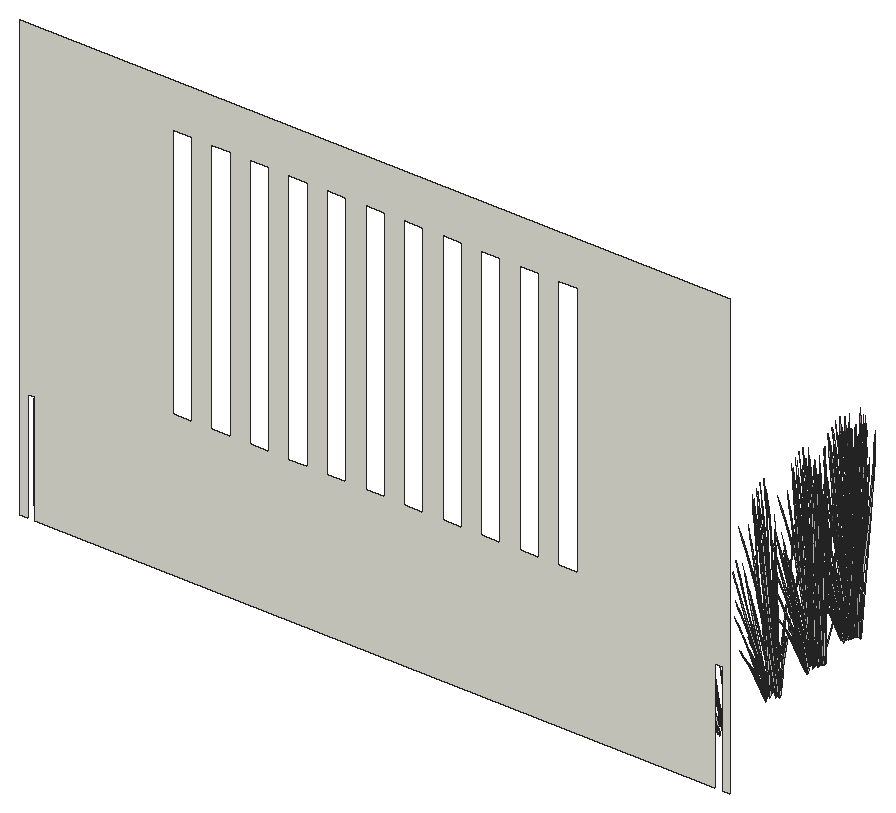
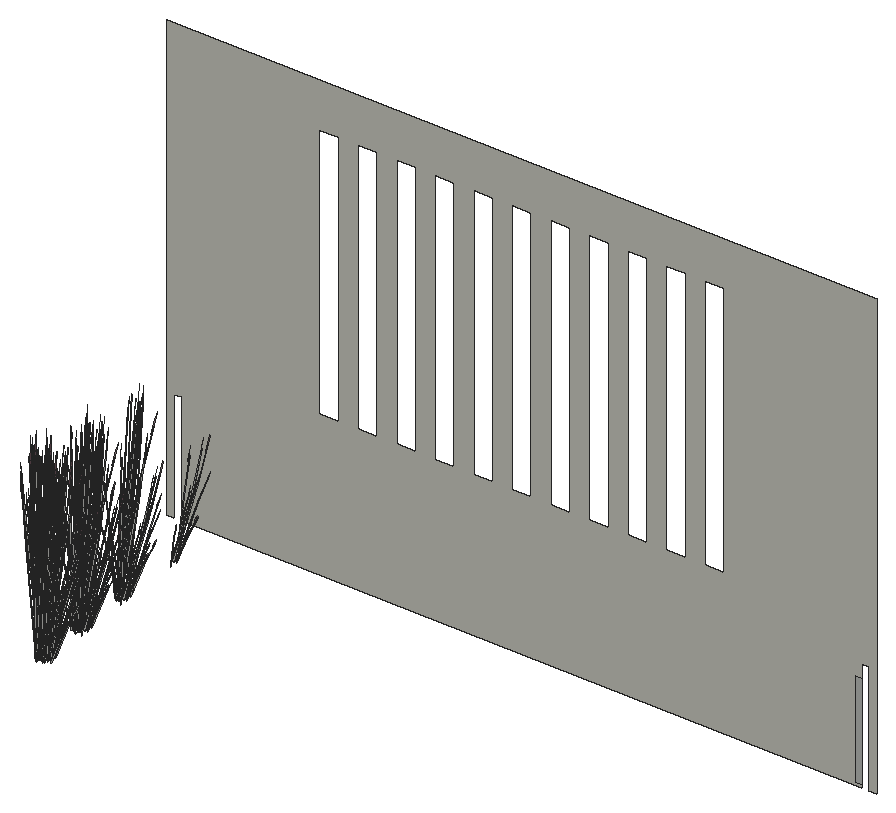
# SketchUp Ruby script. Lengths in inches.
U = 1.inch
M = Sketchup.active_model
def pt(a) = Geom::Point3d.new(a.map { |v| v * U })
def face(e, loops, mat)
  f = e.add_face(loops[0].map { |a| pt(a) })
  loops[1..].each { |l| e.add_face(l.map { |a| pt(a) }).erase! }
  f.material = f.back_material = mat if mat
  f
end
# faces: each face lists its corners as indices into pts; further lists are holes
def faces(e, pts, list, mat = nil) = list.each { |f| face(e, (f[0].is_a?(Array) ? f : [f]).map { |l| l.map { |i| pts[i] } }, mat) }
# xy, xz, yz: faces in a plane at the given z, y or x. An outline is a flat list of corners, or four numbers for a rectangle; further outlines are holes
def ring(l) = l.size == 4 ? [[l[0], l[1]], [l[2], l[1]], [l[2], l[3]], [l[0], l[3]]] : l.each_slice(2).to_a
def flat(e, list, mat, &to3) = list.each { |f| face(e, (f[0].is_a?(Array) ? f : [f]).map { |l| ring(l).map { |u, v| to3.(u, v) } }, mat) }
def xy(e, z, list, mat = nil) = flat(e, list, mat) { |x, y| [x, y, z] }
def xz(e, y, list, mat = nil) = flat(e, list, mat) { |x, z| [x, y, z] }
def yz(e, x, list, mat = nil) = flat(e, list, mat) { |y, z| [x, y, z] }
def lines(e, pts, list) = list.each { |a, b| e.add_line(pt(pts[a]), pt(pts[b])) }
# prism: a flat outline (further loops are holes) pulled along v
def prism(e, loops, v, mat = nil)
  f = face(e, loops, mat); d = Geom::Vector3d.new(v.map { |x| x * U })
  f.pushpull(f.normal.samedirection?(d) ? d.length : -d.length)
end
def box(e, o, s, mat = nil) = prism(e, [[o, [o[0] + s[0], o[1], o[2]], [o[0] + s[0], o[1] + s[1], o[2]], [o[0], o[1] + s[1], o[2]]]], [0, 0, s[2]], mat)
def at(x, y, z, deg = 0) = Geom::Transformation.translation(pt([x, y, z])) * Geom::Transformation.rotation(ORIGIN, Z_AXIS, deg.degrees)
def axes(o, x, y, z) = Geom::Transformation.new([*x, 0, *y, 0, *z, 0, *pt(o).to_a, 1])
def part(name) = M.definitions.add(name)
# library, detail: a bought-in or finely detailed component or shape, given as its bounding box
def library(name, o, s) = part(name).tap { |d| box(d.entities, o, s) }
def detail(e, o, s) = box(e.add_group.entities, o, s)
def put(e, d, t, mat = nil) = e.add_instance(d, t).tap { |i| i.material = mat if mat }
def group(e, t, mat = nil) = e.add_group.tap { |g| g.transformation = t; g.material = mat if mat }.entities
root = M.entities
M.materials.add("D01_Frost_White").color = [238, 238, 227]
M.materials.add("Glass_Basic_01").color = [161, 173, 186]
M.materials["Glass_Basic_01"].alpha = 0.25
M.materials.add("LightPink_Translucent").color = [144, 107, 117]
M.materials["LightPink_Translucent"].alpha = 0.75
c1 = part("blade")
p = [[2.15,0.21,22],[0,0.17,0],[0.09,0.45,0],[2.18,0.31,22],[2.29,0.31,22],[0.38,0.45,0],
  [2.48,0.24,33],[2.49,0.24,33],[2.48,0.22,33]]
faces(c1.entities,p,[[0,1,2,3],[4,5,2,3],[6,3,4,7],[8,0,3,6]])
c2 = part("seeds")
p = [[0.3,-0.1,1.38],[-0.01,-0.03,1.59],[-0.01,-0.03,0.03],[0.14,-0.07,-0.07],[0.29,-0.03,3],[0.15,0.01,3.11]]
faces(c2.entities,p,[[0,1,2,3],[1,0,4,5]],"LightPink_Translucent")
c3 = part("blade with seeds")
put(c3.entities,c1,at(0,0,0))
put(c3.entities,c2,axes([2.4,0.25,30.99],[1.5799,-0.05474,1.17369],[-0.12525,1.92788,0.29478],[-0.07173,-0.02425,1.56792]))
xz(root,178,[[[124,147,124,267,316,267,316,147,314,147,314,177,312,177,312,147,128,147,128,177,126,177,126,147],[269.57,186,274.78,255],[165.22,186,170.43,255],[186.09,186,191.3,255],[196.52,186,201.74,255],[206.96,186,212.17,255],[238.26,186,243.48,255],[248.7,186,253.91,255],[175.65,186,180.87,255],[217.39,186,222.61,255],[227.83,186,233.04,255],[259.13,186,264.35,255]]],"D01_Frost_White")
xz(root,180,[[126,149,128,175]],"Glass_Basic_01")
put(root,c3,axes([300.43,193.49,149.1875],[0.08001,0.13132,1.20808],[-0.18437,0.35694,-0.25981],[-0.18931,-0.08532,0.51652]))
put(root,c3,axes([300.76,193.37,151.21],[-0.40965,-0.01136,-0.60019],[0.02751,-0.47821,0.07243],[-0.17355,-0.05047,0.84903]))
put(root,c3,axes([300.625,193.47,150.95],[-0.29757,0.31243,-0.43168],[-0.2606,-0.33005,-0.33437],[-0.15119,-0.04754,0.82598]))
put(root,c3,axes([299.95,193.88,149.34],[0.26163,-0.03375,0.97034],[-0.16596,0.29737,0.71294],[-0.12929,-0.04461,0.21373]))
put(root,c3,axes([300.14,194.37,148.26],[0.01039,0.07433,1.48974],[-0.20952,0.38819,-0.22758],[-0.14882,-0.01957,0.25375]))
put(root,c3,axes([301.14,194.14,149.82],[0.11649,-0.06823,1.49584],[0.04017,0.47639,0.11706],[-0.25231,0.06321,0.53462]))
put(root,c3,axes([300.34,194.4,150.95],[-0.11102,0.42903,-0.43168],[-0.38064,-0.14706,-0.33437],[-0.15325,0.03934,0.82598]))
put(root,c3,axes([299.88,195.4,149.1875],[0.14242,0.03872,1.20808],[0.09179,0.39548,-0.25981],[-0.19345,0.07403,0.51652]))
put(root,c3,axes([299.58,196.23,149.34],[0.17079,-0.21377,0.97034],[0.06739,0.33841,0.71294],[-0.12342,0.0606,0.21373]))
put(root,c3,axes([300.03,196.45,148.26],[0.05497,0.04712,1.48974],[0.09321,0.43661,-0.22758],[-0.12183,0.0931,0.25375]))
put(root,c3,axes([299.08,211.59,149.1875],[-0.02482,0.15429,1.20808],[-0.36278,0.12916,-0.25981],[-0.0848,-0.19943,0.51652]))
put(root,c3,axes([298.96,211.35,149.34],[0.21377,0.16416,0.97034],[-0.31132,0.09868,0.71294],[-0.06661,-0.12616,0.21373]))
put(root,c3,axes([299.47,212.22,151.21],[-0.34944,-0.22798,-0.60019],[0.24834,-0.39949,0.07243],[-0.1266,-0.13612,0.84903]))
put(root,c3,axes([298.79,211.84,148.26],[-0.0397,0.06213,1.48974],[-0.40116,0.13396,-0.22758],[-0.09691,-0.12186,0.25375]))
put(root,c3,axes([299.31,212.23,150.95],[-0.40438,0.11212,-0.43168],[-0.07074,-0.4246,-0.33437],[-0.10862,-0.12168,0.82598]))
put(root,c3,axes([300.31,214.8,149.81],[0.35414,0.19019,1.27785],[-0.34693,0.40974,0.50532],[-0.1554,-0.24285,1.07126]))
put(root,c3,axes([298.54,212.08,148.8],[-0.11822,0.38513,-0.03288],[-0.36385,-0.11847,-0.1491],[-0.05524,-0.06299,0.4918]))
put(root,c3,axes([298.34,213.84,149],[-0.51243,0,0],[0,-0.52715,-0.43598],[0,-0.12006,1.38303]))
put(root,c3,axes([298.43,212.9,149.1875],[0.08001,0.13132,1.20808],[-0.18437,0.35694,-0.25981],[-0.18931,-0.08532,0.51652]))
put(root,c3,axes([298.76,212.78,151.21],[-0.40965,-0.01136,-0.60019],[0.02751,-0.47821,0.07243],[-0.17355,-0.05047,0.84903]))
put(root,c3,axes([298.74,213.7,148.97],[-0.38118,0.39654,0.25983],[-0.38142,-0.39237,-0.30828],[-0.01331,-0.11261,1.39295]))
put(root,c3,axes([299.77,214.53,149.06],[0.10862,-0.55889,-0.19793],[0.515,0.09742,0.43313],[-0.08999,-0.07718,1.32161]))
put(root,c3,axes([298.625,212.875,150.95],[-0.29757,0.31243,-0.43168],[-0.2606,-0.33005,-0.33437],[-0.15119,-0.04754,0.82598]))
put(root,c3,axes([297.95,213.29,149.34],[0.26163,-0.03375,0.97034],[-0.16596,0.29737,0.71294],[-0.12929,-0.04461,0.21373]))
put(root,c3,axes([299.74,214.3,148.87],[-0.24618,-0.39589,-0.37796],[0.37289,-0.27878,0.1819],[-0.07967,-0.04899,1.2135]))
put(root,c3,axes([299.51,214.45,148.74],[-0.42629,-0.07733,-0.52676],[0.08996,-0.47699,-0.13825],[-0.12722,-0.0578,1.16273]))
put(root,c3,axes([298.14,213.78,148.26],[0.01039,0.07433,1.48974],[-0.20952,0.38819,-0.22758],[-0.14882,-0.01957,0.25375]))
put(root,c3,axes([299.0625,215.18,148.71],[-0.09626,-0.41098,-0.2617],[0.38233,-0.1167,0.2617],[-0.07708,-0.04739,1.17405]))
put(root,c3,axes([298.96,215.35,148.7],[-0.38354,-0.23583,-0.41945],[0.22925,-0.42288,0],[-0.08735,-0.05371,1.33059]))
put(root,c3,axes([300,214.52,149.25],[-0.41376,0.31314,-0.2458],[-0.27514,-0.44246,-0.42242],[-0.10209,-0.04493,1.34921]))
put(root,c3,axes([299.14,213.54,149.82],[0.11649,-0.06823,1.49584],[0.04017,0.47639,0.11706],[-0.25231,0.06321,0.53462]))
put(root,c3,axes([300.46,214.66,149.08],[-0.40016,-0.37963,-0.21282],[0.33672,-0.42629,0.46574],[-0.10776,0.04441,1.42109]))
put(root,c3,axes([299.41,215.39,149.09],[0.38354,0.23583,0.41945],[-0.22925,0.42288,0],[-0.08735,-0.05371,1.33059]))
put(root,c3,axes([298.34,213.8,150.95],[-0.11102,0.42903,-0.43168],[-0.38064,-0.14706,-0.33437],[-0.15325,0.03934,0.82598]))
put(root,c3,axes([299.1875,215.64,149],[-0.25622,0.47263,0],[-0.42866,-0.26357,-0.43598],[-0.09763,-0.06003,1.38303]))
put(root,c3,axes([300.26,214.58,148.87],[-0.44501,0.02912,-0.37796],[-0.04024,-0.48332,0.1819],[-0.07967,0.04899,1.2135]))
put(root,c3,axes([297.88,214.8125,149.1875],[0.14242,0.03872,1.20808],[0.09179,0.39548,-0.25981],[-0.19345,0.07403,0.51652]))
put(root,c3,axes([297.58,215.64,149.34],[0.17079,-0.21377,0.97034],[0.06739,0.33841,0.71294],[-0.12342,0.0606,0.21373]))
put(root,c3,axes([300.27,214.86,148.74],[-0.27603,0.35451,-0.52676],[-0.34289,-0.32147,-0.13825],[-0.11061,0.08844,1.16273]))
put(root,c3,axes([298.52,214.76,150.95],[0.10528,0.43067,-0.43168],[-0.39868,0.07534,-0.33437],[-0.11425,0.11568,0.82598]))
put(root,c3,axes([298.03,215.86,148.26],[0.05497,0.04712,1.48974],[0.09321,0.43661,-0.22758],[-0.12183,0.0931,0.25375]))
put(root,c3,axes([299.03,216.57,149.34],[-0.01061,-0.28045,0.97034],[0.26501,0.20003,0.71294],[-0.05212,0.13367,0.21373]))
put(root,c3,axes([299.04,215.34,151.51],[-0.01066,0.43628,-0.66621],[-0.44902,-0.0293,0.0804],[-0.04739,0.18483,0.94242]))
put(root,c3,axes([298.72,216.32,149.1875],[0.12932,-0.07441,1.20808],[0.31929,0.22435,-0.25981],[-0.09503,0.19413,0.51652]))
put(root,c3,axes([298.89,215.96,149.84],[0.009,-0.24349,1.30391],[0.40497,0.12861,0.18019],[-0.03509,0.2595,0.61571]))
put(root,c3,axes([298.45,227.71,151.21],[-0.19559,-0.38351,-0.60019],[0.40262,-0.21373,0.07243],[-0.04574,-0.1853,0.84903]))
put(root,c3,axes([297.18,227.2,149.1875],[-0.02482,0.15429,1.20808],[-0.36278,0.12916,-0.25981],[-0.0848,-0.19943,0.51652]))
put(root,c3,axes([298.11,226.86,148.26],[-0.06874,0.01699,1.48974],[-0.38012,-0.19128,-0.22758],[0.00638,-0.15955,0.25375]))
put(root,c3,axes([298.3,227.63,150.95],[-0.40284,-0.11824,-0.43168],[0.13808,-0.40538,-0.33437],[-0.03694,-0.16321,0.82598]))
put(root,c3,axes([297.05,226.95,149.34],[0.21377,0.16416,0.97034],[-0.31132,0.09868,0.71294],[-0.06661,-0.12616,0.21373]))
put(root,c3,axes([297.57,227.82,151.21],[-0.34944,-0.22798,-0.60019],[0.24834,-0.39949,0.07243],[-0.1266,-0.13612,0.84903]))
put(root,c3,axes([296.88,227.44,148.26],[-0.0397,0.06213,1.48974],[-0.40116,0.13396,-0.22758],[-0.09691,-0.12186,0.25375]))
put(root,c3,axes([297.55,229.15,148.77],[-0.1683,-0.48366,-0.58997],[0.48479,-0.17419,-0.15484],[-0.0186,-0.16378,1.30225]))
put(root,c3,axes([297.41,227.83,150.95],[-0.40438,0.11212,-0.43168],[-0.07074,-0.4246,-0.33437],[-0.10862,-0.12168,0.82598]))
put(root,c3,axes([298.04,227.19,148.8],[-0.28319,0.27058,-0.03288],[-0.25948,-0.29635,-0.1491],[-0.01827,-0.08397,0.4918]))
put(root,c3,axes([298.41,230.4,149.81],[0.35414,0.19019,1.27785],[-0.34693,0.40974,0.50532],[-0.1554,-0.24285,1.07126]))
put(root,c3,axes([296.55,229.08,148.7],[0,-0.47166,-0.41945],[0.45849,0,0],[0,-0.10742,1.33059]))
put(root,c3,axes([297.8,229.28,148.87],[0.19883,-0.425,-0.37796],[0.41314,0.20454,0.1819],[0,-0.09797,1.2135]))
put(root,c3,axes([296.75,229.09,148.71],[0.28606,-0.29428,-0.2617],[0.28606,0.29428,0.2617],[0,-0.09479,1.17405]))
put(root,c3,axes([296.64,227.68,148.8],[-0.11822,0.38513,-0.03288],[-0.36385,-0.11847,-0.1491],[-0.05524,-0.06299,0.4918]))
put(root,c3,axes([297.75,229.63,149.25],[-0.46151,-0.22505,-0.2458],[0.22222,-0.475,-0.42242],[-0.0145,-0.11662,1.34921]))
put(root,c3,axes([296.44,229.44,149],[-0.51243,0,0],[0,-0.52715,-0.43598],[0,-0.12006,1.38303]))
put(root,c3,axes([296.53,228.5,149.1875],[0.08001,0.13132,1.20808],[-0.18437,0.35694,-0.25981],[-0.18931,-0.08532,0.51652]))
put(root,c3,axes([296.86,228.38,151.21],[-0.40965,-0.01136,-0.60019],[0.02751,-0.47821,0.07243],[-0.17355,-0.05047,0.84903]))
put(root,c3,axes([296.84,229.3,148.97],[-0.38118,0.39654,0.25983],[-0.38142,-0.39237,-0.30828],[-0.01331,-0.11261,1.39295]))
put(root,c3,axes([297.87,230.13,149.06],[0.10862,-0.55889,-0.19793],[0.515,0.09742,0.43313],[-0.08999,-0.07718,1.32161]))
put(root,c3,axes([296.72,228.48,150.95],[-0.29757,0.31243,-0.43168],[-0.2606,-0.33005,-0.33437],[-0.15119,-0.04754,0.82598]))
put(root,c3,axes([296.05,228.89,149.34],[0.26163,-0.03375,0.97034],[-0.16596,0.29737,0.71294],[-0.12929,-0.04461,0.21373]))
put(root,c3,axes([296.75,229.52,149.09],[0,0.47166,0.41945],[-0.45849,0,0],[0,-0.10742,1.33059]))
put(root,c3,axes([297.83,229.9,148.87],[-0.24618,-0.39589,-0.37796],[0.37289,-0.27878,0.1819],[-0.07967,-0.04899,1.2135]))
put(root,c3,axes([297.88,229.34,148.99],[0.17817,0.52741,0.38653],[-0.50909,0.1834,0.15168],[0.00622,-0.09691,1.34202]))
put(root,c3,axes([297.8,229.76,149.3],[-0.19883,0.425,0.37796],[-0.41314,-0.20454,-0.1819],[0,-0.09797,1.2135]))
put(root,c3,axes([297.61,230.05,148.74],[-0.42629,-0.07733,-0.52676],[0.08996,-0.47699,-0.13825],[-0.12722,-0.0578,1.16273]))
put(root,c3,axes([298.65,229.81,148.94],[-0.38118,-0.40596,-0.0518],[0.38142,-0.40621,0],[-0.01331,-0.01418,1.48322]))
put(root,c3,axes([297.93,229.86,148.99],[0.51796,0.09937,0.38653],[-0.10541,0.56124,0.15168],[-0.07569,-0.05419,1.34202]))
put(root,c3,axes([296.24,229.38,148.26],[0.01039,0.07433,1.48974],[-0.20952,0.38819,-0.22758],[-0.14882,-0.01957,0.25375]))
put(root,c3,axes([297.16,230.78,148.71],[-0.09626,-0.41098,-0.2617],[0.38233,-0.1167,0.2617],[-0.07708,-0.04739,1.17405]))
put(root,c3,axes([297.65,230.76,149.09],[0.44036,-0.12519,0.14904],[0.10874,0.46588,0.29641],[-0.03927,-0.06788,1.35512]))
put(root,c3,axes([297.05,230.96,148.7],[-0.38354,-0.23583,-0.41945],[0.22925,-0.42288,0],[-0.08735,-0.05371,1.33059]))
put(root,c3,axes([298.1,230.125,149.25],[-0.41376,0.31314,-0.2458],[-0.27514,-0.44246,-0.42242],[-0.10209,-0.04493,1.34921]))
put(root,c3,axes([298.3125,230.65,148.86],[-0.13371,-0.40664,0],[0.38182,-0.1424,0],[0,0,1.30413]))
put(root,c3,axes([298.06,230.26,149.21],[-0.07906,0.42093,0.12232],[-0.38625,-0.07307,-0.3493],[-0.07029,-0.04322,1.07074]))
put(root,c3,axes([298.96,230.78,149.09],[0.11838,-0.46875,0.14904],[0.43321,0.13265,0.29641],[-0.07483,0.00228,1.35512]))
put(root,c3,axes([297.24,229.15,149.82],[0.11649,-0.06823,1.49584],[0.04017,0.47639,0.11706],[-0.25231,0.06321,0.53462]))
put(root,c3,axes([298.22,230.83,148.86],[-0.41314,-0.21175,0],[0.19883,-0.43999,0],[0,0,1.37455]))
put(root,c3,axes([298.5625,230.27,149.08],[-0.40016,-0.37963,-0.21282],[0.33672,-0.42629,0.46574],[-0.10776,0.04441,1.42109]))
put(root,c3,axes([297.51,230.99,149.09],[0.38354,0.23583,0.41945],[-0.22925,0.42288,0],[-0.08735,-0.05371,1.33059]))
put(root,c3,axes([296.43,229.41,150.95],[-0.11102,0.42903,-0.43168],[-0.38064,-0.14706,-0.33437],[-0.15325,0.03934,0.82598]))
put(root,c3,axes([297.29,231.24,149],[-0.25622,0.47263,0],[-0.42866,-0.26357,-0.43598],[-0.09763,-0.06003,1.38303]))
put(root,c3,axes([298.75,229.95,149.3],[0.44501,-0.02912,0.37796],[0.04024,0.48332,-0.1819],[-0.07967,0.04899,1.2135]))
put(root,c3,axes([298.36,230.1875,148.87],[-0.44501,0.02912,-0.37796],[-0.04024,-0.48332,0.1819],[-0.07967,0.04899,1.2135]))
put(root,c3,axes([298.85,231.31,148.85],[-0.25302,-0.47428,-0.04344],[0.42866,-0.26357,0.43598],[-0.10563,0.04516,1.38235]))
put(root,c3,axes([298.76,230.16,149.21],[0.30276,0.28338,0.12232],[-0.25254,0.31972,-0.3493],[-0.07029,0.04322,1.07074]))
put(root,c3,axes([299.08,231.03,149.09],[0.38354,-0.23583,0.41945],[0.22925,0.42288,0],[-0.08735,0.05371,1.33059]))
put(root,c3,axes([298.74,231.25,148.71],[-0.38233,-0.1167,-0.2617],[0.09626,-0.41098,0.2617],[-0.07708,0.04739,1.17405]))
put(root,c3,axes([295.98,230.41,149.1875],[0.14242,0.03872,1.20808],[0.09179,0.39548,-0.25981],[-0.19345,0.07403,0.51652]))
put(root,c3,axes([295.68,231.24,149.34],[0.17079,-0.21377,0.97034],[0.06739,0.33841,0.71294],[-0.12342,0.0606,0.21373]))
put(root,c3,axes([298.67,230.05,149.25],[0.04775,0.53819,-0.2458],[-0.49736,0.03254,-0.42242],[-0.08758,0.07169,1.34921]))
put(root,c3,axes([298.37,230.47,148.74],[-0.27603,0.35451,-0.52676],[-0.34289,-0.32147,-0.13825],[-0.11061,0.08844,1.16273]))
put(root,c3,axes([298.86,231.0625,148.97],[0.51304,0.1533,0.25983],[-0.12835,0.54797,-0.30828],[-0.08491,0.06858,1.39295]))
put(root,c3,axes([298.83,231.43,148.7],[-0.38354,0.23583,-0.41945],[-0.22925,-0.42288,0],[-0.08735,0.05371,1.33059]))
put(root,c3,axes([296.62,230.36,150.95],[0.10528,0.43067,-0.43168],[-0.39868,0.07534,-0.33437],[-0.11425,0.11568,0.82598]))
put(root,c3,axes([299.17,231.36,149],[0.25622,0.47263,0],[-0.42866,0.26357,-0.43598],[-0.09763,0.06003,1.38303]))
put(root,c3,axes([298.96,229.49,149.4],[-0.01119,-0.44408,1.19347],[0.50665,0.11511,0.50532],[-0.11983,0.243,1.12654]))
put(root,c3,axes([296.13,231.46,148.26],[0.05497,0.04712,1.48974],[0.09321,0.43661,-0.22758],[-0.12183,0.0931,0.25375]))
put(root,c3,axes([297.13,232.17,149.34],[-0.01061,-0.28045,0.97034],[0.26501,0.20003,0.71294],[-0.05212,0.13367,0.21373]))
put(root,c3,axes([297.83,231.5,148.26],[0.06632,-0.02567,1.48974],[0.39894,0.14126,-0.22758],[0.01167,0.15921,0.25375]))
put(root,c3,axes([297.23,231.09,151.23],[0.29336,0.31691,-0.47917],[-0.3099,0.27755,-0.37115],[-0.04464,0.16102,0.91684]))
put(root,c3,axes([296.91,231.57,149.38],[0.37228,-0.08352,0.05498],[0.08559,0.3365,-0.7291],[-0.0236,0.17034,0.65354]))
put(root,c3,axes([297.14,230.95,151.51],[-0.01066,0.43628,-0.66621],[-0.44902,-0.0293,0.0804],[-0.04739,0.18483,0.94242]))
put(root,c3,axes([296.82,231.92,149.1875],[0.12932,-0.07441,1.20808],[0.31929,0.22435,-0.25981],[-0.09503,0.19413,0.51652]))
put(root,c3,axes([296.99,231.5625,149.84],[0.009,-0.24349,1.30391],[0.40497,0.12861,0.18019],[-0.03509,0.2595,0.61571]))
put(root,c3,axes([296.75,242.54,149.1875],[-0.11649,0.09547,1.20808],[-0.34886,-0.1671,-0.25981],[0.06467,-0.20781,0.51652]))
put(root,c3,axes([296.22,242.87,151.21],[-0.19559,-0.38351,-0.60019],[0.40262,-0.21373,0.07243],[-0.04574,-0.1853,0.84903]))
put(root,c3,axes([294.95,242.36,149.1875],[-0.02482,0.15429,1.20808],[-0.36278,0.12916,-0.25981],[-0.0848,-0.19943,0.51652]))
put(root,c3,axes([295.88,242.02,148.26],[-0.06874,0.01699,1.48974],[-0.38012,-0.19128,-0.22758],[0.00638,-0.15955,0.25375]))
put(root,c3,axes([297.03,243.25,151.21],[0.01066,-0.43628,-0.60019],[0.44902,0.0293,0.07243],[0.04739,-0.18483,0.84903]))
put(root,c3,axes([296.07,242.79,150.95],[-0.40284,-0.11824,-0.43168],[0.13808,-0.40538,-0.33437],[-0.03694,-0.16321,0.82598]))
put(root,c3,axes([296.32,241.78,149.34],[0.05257,0.27504,0.97034],[-0.29163,-0.15233,0.71294],[0.03138,-0.14083,0.21373]))
put(root,c3,axes([296.94,243.1,150.95],[-0.29336,-0.31691,-0.43168],[0.3099,-0.27755,-0.33437],[0.04464,-0.16102,0.82598]))
put(root,c3,axes([294.82,242.11,149.34],[0.21377,0.16416,0.97034],[-0.31132,0.09868,0.71294],[-0.06661,-0.12616,0.21373]))
put(root,c3,axes([295.34,242.98,151.21],[-0.34944,-0.22798,-0.60019],[0.24834,-0.39949,0.07243],[-0.1266,-0.13612,0.84903]))
put(root,c3,axes([294.65,242.6,148.26],[-0.0397,0.06213,1.48974],[-0.40116,0.13396,-0.22758],[-0.09691,-0.12186,0.25375]))
put(root,c3,axes([295.32,244.3125,148.77],[-0.1683,-0.48366,-0.58997],[0.48479,-0.17419,-0.15484],[-0.0186,-0.16378,1.30225]))
put(root,c3,axes([295.18,242.99,150.95],[-0.40438,0.11212,-0.43168],[-0.07074,-0.4246,-0.33437],[-0.10862,-0.12168,0.82598]))
put(root,c3,axes([295.25,242.92,149],[-0.25622,-0.47263,0],[0.42866,-0.26357,-0.43598],[0.09763,-0.06003,1.38303]))
put(root,c3,axes([295.8125,242.35,148.8],[-0.28319,0.27058,-0.03288],[-0.25948,-0.29635,-0.1491],[-0.01827,-0.08397,0.4918]))
put(root,c3,axes([296.18,245.56,149.81],[0.35414,0.19019,1.27785],[-0.34693,0.40974,0.50532],[-0.1554,-0.24285,1.07126]))
put(root,c3,axes([294.32,244.24,148.7],[0,-0.47166,-0.41945],[0.45849,0,0],[0,-0.10742,1.33059]))
put(root,c3,axes([295.6,242.85,148.7],[0.38354,-0.23583,-0.41945],[0.22925,0.42288,0],[0.08735,-0.05371,1.33059]))
put(root,c3,axes([295.57,244.4375,148.87],[0.19883,-0.425,-0.37796],[0.41314,0.20454,0.1819],[0,-0.09797,1.2135]))
put(root,c3,axes([295.75,244.23,149.25],[-0.04775,-0.53819,-0.2458],[0.49736,-0.03254,-0.42242],[0.08758,-0.07169,1.34921]))
put(root,c3,axes([294.52,244.25,148.71],[0.28606,-0.29428,-0.2617],[0.28606,0.29428,0.2617],[0,-0.09479,1.17405]))
put(root,c3,axes([294.4,242.84,148.8],[-0.11822,0.38513,-0.03288],[-0.36385,-0.11847,-0.1491],[-0.05524,-0.06299,0.4918]))
put(root,c3,axes([295.52,244.79,149.25],[-0.46151,-0.22505,-0.2458],[0.22222,-0.475,-0.42242],[-0.0145,-0.11662,1.34921]))
put(root,c3,axes([294.21,244.6,149],[-0.51243,0,0],[0,-0.52715,-0.43598],[0,-0.12006,1.38303]))
put(root,c3,axes([294.3,243.66,149.1875],[0.08001,0.13132,1.20808],[-0.18437,0.35694,-0.25981],[-0.18931,-0.08532,0.51652]))
put(root,c3,axes([295.6875,243.03,148.71],[0.38233,0.1167,-0.2617],[-0.09626,0.41098,0.2617],[0.07708,-0.04739,1.17405]))
put(root,c3,axes([294.625,243.54,151.21],[-0.40965,-0.01136,-0.60019],[0.02751,-0.47821,0.07243],[-0.17355,-0.05047,0.84903]))
put(root,c3,axes([294.61,244.46,148.97],[-0.38118,0.39654,0.25983],[-0.38142,-0.39237,-0.30828],[-0.01331,-0.11261,1.39295]))
put(root,c3,axes([295.82,244.65,149.06],[0.46174,0.2286,0.2033],[-0.22222,0.475,0.42242],[0,-0.1095,1.35626]))
put(root,c3,axes([295.64,245.29,149.06],[0.10862,-0.55889,-0.19793],[0.515,0.09742,0.43313],[-0.08999,-0.07718,1.32161]))
put(root,c3,axes([294.49,243.64,150.95],[-0.29757,0.31243,-0.43168],[-0.2606,-0.33005,-0.33437],[-0.15119,-0.04754,0.82598]))
put(root,c3,axes([293.82,244.05,149.34],[0.26163,-0.03375,0.97034],[-0.16596,0.29737,0.71294],[-0.12929,-0.04461,0.21373]))
put(root,c3,axes([295.67,244.33,149.3],[-0.44501,0.02912,0.37796],[-0.04024,-0.48332,-0.1819],[0.07967,-0.04899,1.2135]))
put(root,c3,axes([294.52,244.68,149.09],[0,0.47166,0.41945],[-0.45849,0,0],[0,-0.10742,1.33059]))
put(root,c3,axes([295.6,245.0625,148.87],[-0.24618,-0.39589,-0.37796],[0.37289,-0.27878,0.1819],[-0.07967,-0.04899,1.2135]))
put(root,c3,axes([295.65,244.5,148.99],[0.17817,0.52741,0.38653],[-0.50909,0.1834,0.15168],[0.00622,-0.09691,1.34202]))
put(root,c3,axes([295.5625,244.92,149.3],[-0.19883,0.425,0.37796],[-0.41314,-0.20454,-0.1819],[0,-0.09797,1.2135]))
put(root,c3,axes([296.29,244.55,148.86],[0,-0.54574,0],[0.51243,0,0],[0,0,1.51605]))
put(root,c3,axes([296.92,243.29,149.09],[-0.38354,-0.23583,0.41945],[0.22925,-0.42288,0],[0.08735,0.05371,1.33059]))
put(root,c3,axes([295.38,245.21,148.74],[-0.42629,-0.07733,-0.52676],[0.08996,-0.47699,-0.13825],[-0.12722,-0.0578,1.16273]))
put(root,c3,axes([296.05,244.2,148.99],[-0.33979,0.42804,0.38653],[-0.40368,-0.37784,0.15168],[0.08192,-0.04272,1.34202]))
put(root,c3,axes([296.42,244.97,148.94],[-0.38118,-0.40596,-0.0518],[0.38142,-0.40621,0],[-0.01331,-0.01418,1.48322]))
put(root,c3,axes([295.46,243.5,149.09],[-0.11838,0.46875,0.14904],[-0.43321,-0.13265,0.29641],[0.07483,-0.00228,1.35512]))
put(root,c3,axes([296.37,244.02,149.21],[0.07906,-0.42093,0.12232],[0.38625,0.07307,-0.3493],[0.07029,0.04322,1.07074]))
put(root,c3,axes([295.7,245.02,148.99],[0.51796,0.09937,0.38653],[-0.10541,0.56124,0.15168],[-0.07569,-0.05419,1.34202]))
put(root,c3,axes([294.01,244.54,148.26],[0.01039,0.07433,1.48974],[-0.20952,0.38819,-0.22758],[-0.14882,-0.01957,0.25375]))
put(root,c3,axes([296.2,244.13,149.3],[-0.24618,-0.39589,0.37796],[0.37289,-0.27878,-0.1819],[0.07967,0.04899,1.2135]))
put(root,c3,axes([294.93,245.94,148.71],[-0.09626,-0.41098,-0.2617],[0.38233,-0.1167,0.2617],[-0.07708,-0.04739,1.17405]))
put(root,c3,axes([295.42,245.92,149.09],[0.44036,-0.12519,0.14904],[0.10874,0.46588,0.29641],[-0.03927,-0.06788,1.35512]))
put(root,c3,axes([294.82,246.12,148.7],[-0.38354,-0.23583,-0.41945],[0.22925,-0.42288,0],[-0.08735,-0.05371,1.33059]))
put(root,c3,axes([293.97,244.37,150.82],[-0.34057,-0.13158,-0.29918],[0.09933,-0.38387,0.38624],[-0.13712,0.0352,0.73904]))
put(root,c3,axes([296.64,244.67,148.86],[0.45849,0,0],[0,0.4883,0],[0,0,1.50718]))
put(root,c3,axes([295.87,245.29,149.25],[-0.41376,0.31314,-0.2458],[-0.27514,-0.44246,-0.42242],[-0.10209,-0.04493,1.34921]))
put(root,c3,axes([296.77,243.53,149.09],[-0.44036,0.12519,0.14904],[-0.10874,-0.46588,0.29641],[0.03927,0.06788,1.35512]))
put(root,c3,axes([296.49,244.42,149.01],[-0.51796,-0.09937,0.41563],[0.10541,-0.56124,0.1631],[0.07569,0.05419,1.44303]))
put(root,c3,axes([296.08,245.81,148.86],[-0.13371,-0.40664,0],[0.38182,-0.1424,0],[0,0,1.30413]))
put(root,c3,axes([295.83,245.42,149.21],[-0.07906,0.42093,0.12232],[-0.38625,-0.07307,-0.3493],[-0.07029,-0.04322,1.07074]))
put(root,c3,axes([296.58,245.75,148.85],[0.43024,-0.16003,-0.16218],[0.15118,0.46099,0.00007],[0.04749,-0.01769,1.46908]))
put(root,c3,axes([296.73,245.94,149.09],[0.11838,-0.46875,0.14904],[0.43321,0.13265,0.29641],[-0.07483,0.00228,1.35512]))
put(root,c3,axes([296.63,244.88,148.87],[0.28606,0.30466,0],[-0.28606,0.30466,0],[0,0,1.42996]))
put(root,c3,axes([295.01,244.31,149.82],[0.11649,-0.06823,1.49584],[0.04017,0.47639,0.11706],[-0.25231,0.06321,0.53462]))
put(root,c3,axes([297.41,244.75,149.09],[-0.32198,-0.34356,0.14904],[0.32447,-0.33323,0.29641],[-0.03556,0.07016,1.35512]))
put(root,c3,axes([295.99,245.99,148.86],[-0.41314,-0.21175,0],[0.19883,-0.43999,0],[0,0,1.37455]))
put(root,c3,axes([296.33,245.43,149.08],[-0.40016,-0.37963,-0.21282],[0.33672,-0.42629,0.46574],[-0.10776,0.04441,1.42109]))
put(root,c3,axes([295.28,246.16,149.09],[0.38354,0.23583,0.41945],[-0.22925,0.42288,0],[-0.08735,-0.05371,1.33059]))
put(root,c3,axes([296.63,244.52,149.3],[0.19883,-0.425,0.37796],[0.41314,0.20454,-0.1819],[0,0.09797,1.2135]))
put(root,c3,axes([296.55,244.77,148.9375],[0,0.54548,-0.04762],[-0.51243,0,0],[0,0.01714,1.5153]))
put(root,c3,axes([294.2,244.57,150.95],[-0.11102,0.42903,-0.43168],[-0.38064,-0.14706,-0.33437],[-0.15325,0.03934,0.82598]))
put(root,c3,axes([296.59,244.38,148.87],[0.24618,0.39589,-0.37796],[-0.37289,0.27878,0.1819],[0.07967,0.04899,1.2135]))
put(root,c3,axes([295.06,246.4,149],[-0.25622,0.47263,0],[-0.42866,-0.26357,-0.43598],[-0.09763,-0.06003,1.38303]))
put(root,c3,axes([297.67,244.76,149.09],[0,-0.47166,0.41945],[0.45849,0,0],[0,0.10742,1.33059]))
put(root,c3,axes([296.52,245.11,149.3],[0.44501,-0.02912,0.37796],[0.04024,0.48332,-0.1819],[-0.07967,0.04899,1.2135]))
put(root,c3,axes([296.8,244.62,149.21],[0.38182,-0.13755,0.12232],[0.13371,0.39278,-0.3493],[0,0.08644,1.07074]))
put(root,c3,axes([296.13,245.35,148.87],[-0.44501,0.02912,-0.37796],[-0.04024,-0.48332,0.1819],[-0.07967,0.04899,1.2135]))
put(root,c3,axes([296.46,246,148.86],[0.41314,0.21175,0],[-0.19883,0.43999,0],[0,0,1.47801]))
put(root,c3,axes([296.62,246.47,148.85],[-0.25302,-0.47428,-0.04344],[0.42866,-0.26357,0.43598],[-0.10563,0.04516,1.38235]))
put(root,c3,axes([296.53,245.32,149.21],[0.30276,0.28338,0.12232],[-0.25254,0.31972,-0.3493],[-0.07029,0.04322,1.07074]))
put(root,c3,axes([296.85,246.19,149.09],[0.38354,-0.23583,0.41945],[0.22925,0.42288,0],[-0.08735,0.05371,1.33059]))
put(root,c3,axes([296.31,245.82,148.9375],[0.17817,0.54185,-0.05079],[-0.50909,0.18987,0],[0.00622,0.01892,1.45452]))
put(root,c3,axes([296.5,246.41,148.71],[-0.38233,-0.1167,-0.2617],[0.09626,-0.41098,0.2617],[-0.07708,0.04739,1.17405]))
put(root,c3,axes([293.75,245.57,149.1875],[0.14242,0.03872,1.20808],[0.09179,0.39548,-0.25981],[-0.19345,0.07403,0.51652]))
put(root,c3,axes([297.78,245.11,148.86],[-0.51218,-0.00377,-0.04204],[0,-0.52715,0.42192],[-0.0161,0.12,1.33776]))
put(root,c3,axes([296.67,244.65,149.25],[0.46151,0.22505,-0.2458],[-0.22222,0.475,-0.42242],[0.0145,0.11662,1.34921]))
put(root,c3,axes([293.45,246.4,149.34],[0.17079,-0.21377,0.97034],[0.06739,0.33841,0.71294],[-0.12342,0.0606,0.21373]))
put(root,c3,axes([297.67,245.1875,148.71],[-0.28606,0.29428,-0.2617],[-0.28606,-0.29428,0.2617],[0,0.09479,1.17405]))
put(root,c3,axes([296.4375,245.22,149.25],[0.04775,0.53819,-0.2458],[-0.49736,0.03254,-0.42242],[-0.08758,0.07169,1.34921]))
put(root,c3,axes([296.62,245.01,148.87],[-0.19883,0.425,-0.37796],[-0.41314,-0.20454,0.1819],[0,0.09797,1.2135]))
put(root,c3,axes([296.14,245.625,148.74],[-0.27603,0.35451,-0.52676],[-0.34289,-0.32147,-0.13825],[-0.11061,0.08844,1.16273]))
put(root,c3,axes([296.63,246.22,148.97],[0.51304,0.1533,0.25983],[-0.12835,0.54797,-0.30828],[-0.08491,0.06858,1.39295]))
put(root,c3,axes([296.59,246.59,148.7],[-0.38354,0.23583,-0.41945],[-0.22925,-0.42288,0],[-0.08735,0.05371,1.33059]))
put(root,c3,axes([297.87,245.2,148.7],[0,0.47166,-0.41945],[-0.45849,0,0],[0,0.10742,1.33059]))
put(root,c3,axes([294.39,245.52,150.95],[0.10528,0.43067,-0.43168],[-0.39868,0.07534,-0.33437],[-0.11425,0.11568,0.82598]))
